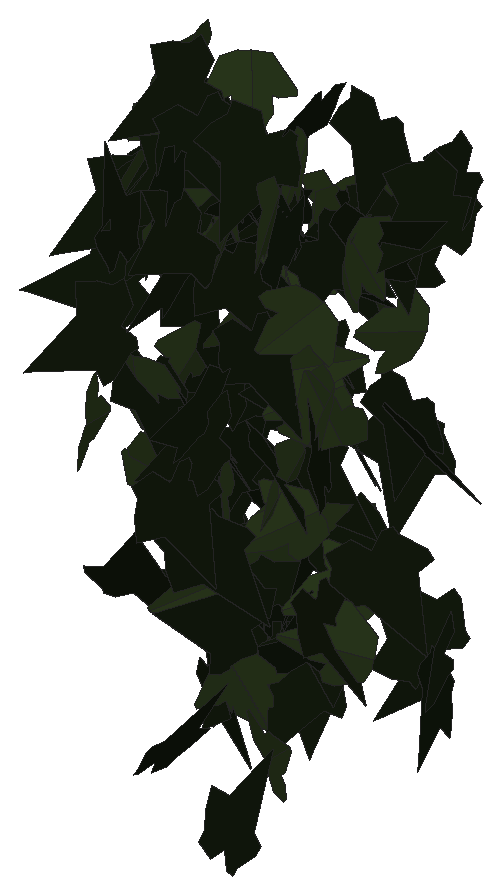
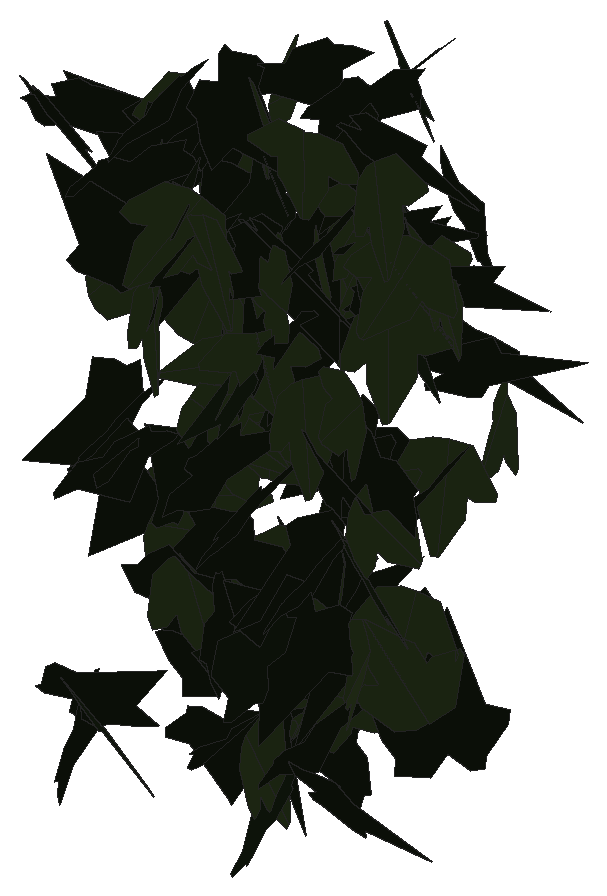
# SketchUp Ruby script. Lengths in inches.
U = 1.inch
M = Sketchup.active_model
def pt(a) = Geom::Point3d.new(a.map { |v| v * U })
def face(e, loops, mat)
  f = e.add_face(loops[0].map { |a| pt(a) })
  loops[1..].each { |l| e.add_face(l.map { |a| pt(a) }).erase! }
  f.material = f.back_material = mat if mat
  f
end
# faces: each face lists its corners as indices into pts; further lists are holes
def faces(e, pts, list, mat = nil) = list.each { |f| face(e, (f[0].is_a?(Array) ? f : [f]).map { |l| l.map { |i| pts[i] } }, mat) }
# xy, xz, yz: faces in a plane at the given z, y or x. An outline is a flat list of corners, or four numbers for a rectangle; further outlines are holes
def ring(l) = l.size == 4 ? [[l[0], l[1]], [l[2], l[1]], [l[2], l[3]], [l[0], l[3]]] : l.each_slice(2).to_a
def flat(e, list, mat, &to3) = list.each { |f| face(e, (f[0].is_a?(Array) ? f : [f]).map { |l| ring(l).map { |u, v| to3.(u, v) } }, mat) }
def xy(e, z, list, mat = nil) = flat(e, list, mat) { |x, y| [x, y, z] }
def xz(e, y, list, mat = nil) = flat(e, list, mat) { |x, z| [x, y, z] }
def yz(e, x, list, mat = nil) = flat(e, list, mat) { |y, z| [x, y, z] }
def lines(e, pts, list) = list.each { |a, b| e.add_line(pt(pts[a]), pt(pts[b])) }
# prism: a flat outline (further loops are holes) pulled along v
def prism(e, loops, v, mat = nil)
  f = face(e, loops, mat); d = Geom::Vector3d.new(v.map { |x| x * U })
  f.pushpull(f.normal.samedirection?(d) ? d.length : -d.length)
end
def box(e, o, s, mat = nil) = prism(e, [[o, [o[0] + s[0], o[1], o[2]], [o[0] + s[0], o[1] + s[1], o[2]], [o[0], o[1] + s[1], o[2]]]], [0, 0, s[2]], mat)
def at(x, y, z, deg = 0) = Geom::Transformation.translation(pt([x, y, z])) * Geom::Transformation.rotation(ORIGIN, Z_AXIS, deg.degrees)
def axes(o, x, y, z) = Geom::Transformation.new([*x, 0, *y, 0, *z, 0, *pt(o).to_a, 1])
def part(name) = M.definitions.add(name)
# library, detail: a bought-in or finely detailed component or shape, given as its bounding box
def library(name, o, s) = part(name).tap { |d| box(d.entities, o, s) }
def detail(e, o, s) = box(e.add_group.entities, o, s)
def put(e, d, t, mat = nil) = e.add_instance(d, t).tap { |i| i.material = mat if mat }
def group(e, t, mat = nil) = e.add_group.tap { |g| g.transformation = t; g.material = mat if mat }.entities
root = M.entities
M.materials.add("efeu1").color = [18, 25, 13]
M.materials.add("efeu2").color = [43, 57, 29]
c1 = part("ivyleaf_9")
p = [[1.54,2.16,1.25],[1.36,2.04,1.19],[-0.21,0.99,0.68],[-0.71,1.11,0.82],[-0.85,0.86,0.67],[-0.8,0.17,0.21],
  [-0.9,-0.01,0.1],[-0.67,-0.16,-0.02],[-0.08,-0.08,-0.05],[-0.03,-0.6,-0.4],[0.65,-0.88,-0.66],[0.83,-0.6,-0.49],
  [1.29,-0.42,-0.43],[1.8125,-0.07,-0.26],[1.21,0.44,0.15]]
faces(c1.entities,p,[[0,1,2,3,4,5,6,7,8,9,10,11,12,13,14]],"efeu1")
c2 = part("ivyleaf_10")
p = [[0,0.5,-0.03],[-0.0625,2.02,-0.43],[-0.19,2.01,-0.46],[-0.54,1.05,-0.29],[-0.52,0.625,-0.18],[-0.83,0.76,-0.28],
  [-1.16,0.64,-0.33],[-1.15,0.33,-0.24],[-0.77,-0.39,0.02],[-0.3,-0.51,0.16],[0.04,-0.48,0.23],[-0.02,2.01,-0.4375],
  [-0.06,2.01,-0.43],[0.04,-0.49,0.23],[0.67,-0.49,0.14],[1.38,0.36,-0.2],[1.375,0.51,-0.24],[0.81,0.65,-0.19],
  [0.62,0.59,-0.15],[0.6,1.09,-0.28],[0.5,1.23,-0.31]]
faces(c2.entities,p,[[0,1,2,3,4,5,6,7,8,9,10],[11,12,0,13,14,15,16,17,18,19,20]],"efeu2")
put(root,c1,axes([44.17,216.95,233.36],[-0.29201,0.31391,0.25727],[0.16965,-0.19353,0.42868],[0.36872,0.33765,0.00651]))
put(root,c1,axes([43.1875,217.07,238.26],[0.09081,-0.40776,-0.27475],[-0.05016,0.27025,-0.41767],[0.48912,0.10342,0.00818]))
put(root,c1,axes([43.4,217.47,239.27],[-0.33404,0.36237,0.08429],[-0.06458,0.05508,-0.49274],[-0.3664,-0.34008,0.01001]))
put(root,c1,axes([43.44,217.63,238.82],[-0.46053,0.16691,0.10026],[-0.09211,0.04007,-0.48981],[-0.17154,-0.46961,-0.00615]))
put(root,c1,axes([42.54,217.61,233.78],[0.12144,0.48134,0.0597],[-0.01468,-0.05787,0.49642],[0.48481,-0.12232,0.00007]))
put(root,c1,axes([42.3,218.62,241.02],[-0.23644,-0.26405,0.35267],[-0.0424,-0.38475,-0.3165],[0.43852,-0.17957,0.15955]))
put(root,c1,axes([42.65,218.31,236.78],[-0.0992,-0.12338,-0.47427],[0.29676,0.36996,-0.15831],[0.38999,-0.3129,-0.00017]))
put(root,c1,axes([41.8125,218.78,241.72],[-0.30616,0.00311,-0.3953],[0.38456,-0.11348,-0.29873],[-0.09157,-0.48694,0.06709]))
put(root,c2,axes([43.38,218.8,233.52],[-0.31281,0.08218,0.38131],[0.36576,-0.10801,0.32334],[0.13552,0.48123,0.00746]))
put(root,c2,axes([44.71,218.92,235.52],[0.06726,0.05582,0.4923],[-0.38955,-0.30103,0.08735],[0.30615,-0.3953,0.003]))
put(root,c2,axes([40.68,218.45,237.75],[0.03733,-0.19459,-0.45906],[-0.06731,0.45417,-0.19799],[0.49404,0.07658,0.00771]))
put(root,c1,axes([44.1875,218.84,236.09],[0.26012,-0.38428,-0.18619],[-0.10089,0.15654,-0.46402],[0.41492,0.27898,0.0039]))
put(root,c1,axes([40.67,219.06,238.86],[-0.47798,0.04874,0.13844],[-0.13878,0.00338,-0.48034],[-0.04776,-0.49761,0.01029]))
put(root,c1,axes([41.76,219.1,240.16],[-0.39385,0.2937,-0.09287],[0.07562,-0.05394,-0.4913],[-0.29861,-0.40104,-0.00193]))
put(root,c1,axes([42.52,219.4375,234.9],[-0.07693,-0.05425,0.49106],[-0.3839,-0.30625,-0.09398],[0.31097,-0.39149,0.00547]))
put(root,c1,axes([40.82,218.93,240.1875],[0.08447,0.03015,0.49189],[-0.20318,0.4568,0.00689],[-0.44898,-0.20105,0.08942]))
put(root,c2,axes([42.86,219.51,241.18],[0.05398,-0.15015,0.47386],[0.30302,-0.3679,-0.15109],[0.39404,0.30349,0.05128]))
put(root,c2,axes([43.4375,219.42,236.86],[-0.18949,-0.12269,0.44614],[-0.2797,-0.35368,-0.21605],[0.3686,-0.33145,0.0654]))
put(root,c1,axes([42.73,219.3,239.34],[-0.17253,-0.1136,-0.45533],[0.37118,0.26382,-0.20646],[0.28716,-0.40926,-0.0067]))
put(root,c2,axes([43.58,219.37,239.95],[0.36612,0.07803,-0.33146],[-0.33824,0.02713,-0.36723],[-0.03933,0.49313,0.07266]))
put(root,c2,axes([43.04,219.73,237.35],[0.08516,-0.18325,0.45735],[0.2054,-0.40867,-0.202],[0.44784,0.22228,0.00567]))
put(root,c2,axes([42.52,219.28,234.26],[-0.32308,-0.33079,-0.19025],[0.1444,0.12477,-0.46215],[0.35323,-0.35356,0.01491]))
put(root,c1,axes([43.84,219.36,237.59],[0.09451,-0.36638,0.32686],[0.04105,0.33759,0.36653],[-0.48927,-0.04245,0.0939]))
put(root,c1,axes([42.8,219.68,237.4],[0.15539,-0.3737,0.2936],[0.1732,-0.24313,-0.40111],[0.44256,0.22636,0.05389]))
put(root,c2,axes([43.88,219.54,238.23],[-0.43634,-0.16803,-0.17712],[-0.16603,-0.06174,0.46757],[-0.17901,0.46685,-0.00191]))
put(root,c2,axes([43.81,219.42,238.79],[0.32451,-0.34146,-0.16763],[-0.11759,0.1195,-0.47105],[0.36175,0.34515,-0.00275]))
put(root,c1,axes([41.76,219.63,233.9],[-0.0089,0.01269,-0.49976],[0.499,0.03056,-0.00811],[0.03033,-0.4989,-0.0132]))
put(root,c1,axes([42.46,219.86,241.93],[-0.27279,-0.41886,0.01203],[-0.00827,-0.00898,-0.49985],[0.41895,-0.27291,-0.00203]))
put(root,c1,axes([40.26,219.91,239.02],[-0.33135,-0.04916,0.3712],[-0.33074,-0.19397,-0.32092],[0.17556,-0.45821,0.09602]))
put(root,c2,axes([43.96,219.93,235.82],[-0.18203,0.01179,0.46554],[-0.23954,-0.43102,-0.08274],[0.39936,-0.25315,0.16256]))
put(root,c1,axes([41.49,219.73,241.91],[0.0202,-0.39898,-0.30068],[0.0152,0.30128,-0.39875],[0.49936,0.00697,0.0243]))
put(root,c1,axes([40.3,219.89,234.48],[0.47165,0.05631,0.15613],[-0.15478,-0.02058,0.475],[0.05992,-0.49639,-0.00198]))
put(root,c1,axes([43.16,219.89,234.47],[0.38109,0.21726,0.23993],[-0.2205,-0.09709,0.43813],[0.23696,-0.43974,0.02181]))
put(root,c1,axes([41.52,219.65,237.61],[0.45763,-0.04302,-0.19678],[-0.19307,0.04556,-0.45896],[0.05742,0.49606,0.02509]))
put(root,c1,axes([42.125,220.24,233.93],[-0.17309,-0.36371,0.29623],[-0.08076,-0.28793,-0.40071],[0.46208,-0.18657,0.04093]))
put(root,c2,axes([40.41,219.82,237.83],[-0.49301,-0.07431,0.03763],[-0.03669,-0.00909,-0.49857],[0.07479,-0.49436,0.00351]))
put(root,c1,axes([43.02,219.55,240.46],[-0.01399,0.16256,0.47263],[-0.16266,0.4456,-0.15807],[-0.4726,-0.15818,0.04041]))
put(root,c1,axes([40.29,220.17,240.17],[-0.40828,-0.20075,0.20738],[-0.15858,-0.14415,-0.45174],[0.24117,-0.43465,0.05404]))
put(root,c2,axes([41.58,220.13,236.375],[-0.17197,0.17532,-0.43554],[0.20308,-0.39042,-0.23734],[-0.4233,-0.25852,0.06307]))
put(root,c1,axes([40.4,220.09,237.64],[0.11712,-0.48603,-0.00796],[-0.00042,0.00808,-0.49993],[0.48609,0.11711,0.00148]))
put(root,c2,axes([44.125,219.74,240.92],[-0.0946,0.42249,0.2501],[-0.09576,0.23393,-0.4314],[-0.48154,-0.12952,0.03665]))
put(root,c1,axes([44.17,219.99,236.31],[-0.08439,-0.30346,-0.38832],[0.2181,0.33029,-0.30552],[0.44194,-0.22095,0.07662]))
put(root,c1,axes([40.95,220.37,240.6],[-0.34879,-0.23503,0.27038],[-0.16878,-0.22506,-0.41336],[0.31601,-0.37962,0.07766]))
put(root,c2,axes([40.98,219.81,240.24],[-0.15524,-0.31879,-0.35252],[0.23607,0.27015,-0.34826],[0.41252,-0.27457,0.06664]))
put(root,c2,axes([44.05,219.6875,240.66],[-0.06117,0.21059,0.44935],[-0.27302,0.36379,-0.20765],[-0.41439,-0.27076,0.07049]))
put(root,c2,axes([41.49,220.25,234.875],[0.14082,0.14904,-0.45602],[-0.39655,-0.23134,-0.19807],[-0.27003,0.41745,0.05305]))
put(root,c1,axes([41.32,219.95,241.375],[0.47809,-0.07001,-0.12857],[-0.12677,0.02164,-0.48318],[0.07322,0.4946,0.00294]))
put(root,c2,axes([41.59,220.26,240.29],[0.14256,-0.4602,0.13378],[0.0301,-0.1307,-0.48168],[0.4783,0.14539,-0.00956]))
put(root,c1,axes([43.43,219.85,240.74],[0.1524,-0.17094,-0.44447],[-0.14093,0.42958,-0.21354],[0.45488,0.19036,0.08276]))
put(root,c1,axes([42.76,220.47,233.98],[-0.2178,-0.43133,0.12852],[-0.00011,-0.14273,-0.4792],[0.45007,-0.20876,0.06207]))
put(root,c2,axes([40.45,220.23,240.69],[0.40656,-0.28415,0.06299],[0.05167,-0.03603,-0.49602],[0.28643,0.40983,0.00007]))
put(root,c2,axes([42.7,220.36,239.27],[0.10063,-0.45376,0.18433],[0.02622,-0.18291,-0.4646],[0.48907,0.10317,-0.01302]))
put(root,c2,axes([42.76,220.18,241.68],[0.36785,-0.32655,-0.0897],[-0.05342,0.07483,-0.49147],[0.33441,0.37117,0.02017]))
put(root,c2,axes([42.33,219.97,236.07],[-0.23647,-0.24217,-0.36802],[0.24327,0.27645,-0.33822],[0.36729,-0.33901,-0.01292]))
put(root,c1,axes([40.49,220.55,240.29],[-0.31565,-0.38671,0.02865],[-0.0178,-0.02246,-0.49918],[0.38736,-0.31615,0.00042]))
put(root,c2,axes([40,220.42,240.53],[0.15917,-0.47138,0.04967],[0.01528,-0.04726,-0.49753],[0.47374,0.1599,-0.00065]))
put(root,c1,axes([40.9,220.48,241.92],[-0.49003,-0.00936,0.09889],[-0.0986,-0.01438,-0.48997],[0.01202,-0.49971,0.01225]))
put(root,c1,axes([43.73,220.29,240.49],[0.01571,-0.09515,0.49061],[0.48872,-0.09964,-0.03497],[0.10443,0.48064,0.08987]))
put(root,c1,axes([42.05,220.65,235.26],[-0.43503,-0.24229,0.04517],[-0.04097,-0.01927,-0.49795],[0.24304,-0.43695,-0.00309]))
put(root,c1,axes([42.67,220.3125,240.1],[0.4275,-0.05709,0.25295],[0.249,-0.04579,-0.43116],[0.07239,0.49462,-0.01072]))
put(root,c1,axes([42.13,220.4,240.72],[0.44565,-0.22128,0.04925],[0.04367,-0.02279,-0.49757],[0.22245,0.44779,-0.00099]))
put(root,c1,axes([42.74,220.56,234.21],[-0.29414,-0.32896,-0.23509],[0.14938,0.18174,-0.4412],[0.37572,-0.32979,-0.00864]))
put(root,c1,axes([40.85,220.37,240.16],[-0.32289,0.38042,-0.03191],[0.02019,-0.02473,-0.49898],[-0.38122,-0.32352,0.00061]))
put(root,c2,axes([41.11,220.45,240.78],[-0.4075,0.21224,-0.19723],[0.1653,-0.10922,-0.45907],[-0.23795,-0.43935,0.01884]))
put(root,c2,axes([42.71,220.15,238.43],[0.00134,-0.03376,0.49886],[0.1628,0.4717,0.03149],[-0.47275,0.16235,0.01225]))
put(root,c2,axes([40.375,220.47,236.31],[-0.49363,-0.06856,-0.04031],[0.04018,0.00373,-0.49837],[0.06863,-0.49526,0.00183]))
put(root,c2,axes([44.05,220.87,239.19],[-0.01322,0.19339,0.4609],[0.05102,-0.45813,0.19369],[0.49721,0.05215,-0.00762]))
put(root,c2,axes([40.7,220.43,240.07],[-0.34681,0.08061,0.35104],[-0.347,0.05582,-0.35563],[-0.09652,-0.49029,0.01722]))
put(root,c1,axes([41.11,220.44,235.73],[0.15677,-0.32778,-0.34349],[-0.15226,0.30792,-0.36332],[0.44971,0.21851,-0.00327]))
put(root,c2,axes([42.85,220.73,237.95],[-0.24859,0.00617,0.43378],[-0.37312,-0.25809,-0.21016],[0.22132,-0.42819,0.13292]))
put(root,c1,axes([41.49,220.25,236.69],[0.07045,0.01906,-0.49464],[-0.13744,0.48074,-0.00105],[0.47555,0.13611,0.07298]))
put(root,c2,axes([42.23,220.97,238.59],[0.05508,0.16523,-0.46868],[-0.13327,-0.44937,-0.17409],[-0.47875,0.1441,-0.00546]))
put(root,c1,axes([41.4,220.59,239.47],[0.01739,-0.36795,-0.33809],[-0.02266,0.33737,-0.36833],[0.49918,0.02814,-0.00495]))
put(root,c1,axes([42.59,220.82,242.04],[-0.22735,0.2606,-0.36111],[0.18797,-0.31141,-0.34306],[-0.40371,-0.29175,0.04363]))
put(root,c1,axes([42.53,220.97,235.78],[-0.1274,0.03761,-0.48203],[0.37614,-0.3055,-0.12325],[-0.30379,-0.39402,0.04955]))
put(root,c1,axes([41.82,220.66,240.45],[0.064,0.38027,-0.31827],[-0.10249,-0.30384,-0.38364],[-0.48518,0.11434,0.03906]))
put(root,c2,axes([40.46,220.97,237.71],[-0.01193,-0.38616,0.31739],[0.02091,-0.31759,-0.38562],[0.49942,0.00408,0.02373]))
put(root,c1,axes([42.1,220.99,238.74],[-0.01282,-0.07901,0.49355],[0.12935,-0.47742,-0.07307],[0.48281,0.12581,0.03268]))
put(root,c1,axes([41.53,220.57,237.69],[-0.33788,0.0425,-0.36611],[-0.368,-0.01142,0.3383],[0.0204,0.49806,0.039]))
put(root,c1,axes([43.34,220.8,235.5625],[-0.14754,0.05781,0.47423],[-0.46365,0.10232,-0.15672],[-0.11516,-0.48599,0.02342]))
put(root,c1,axes([42.08,220.59,234.63],[0.06388,-0.00337,-0.49589],[-0.49571,0.0136,-0.06395],[0.01392,0.4998,-0.0016]))
put(root,c1,axes([42.92,221.02,237.24],[0.16407,-0.2583,0.39543],[0.19077,-0.3467,-0.30563],[0.43207,0.25116,-0.01521]))
put(root,c2,axes([40.31,220.45,240.09],[0.14963,0.23983,0.41242],[0.11632,0.40085,-0.2753],[-0.46269,0.17833,0.06417]))
put(root,c1,axes([44.57,221.03,241.29],[-0.44056,-0.22312,0.07825],[-0.06274,-0.04924,-0.4936],[0.22797,-0.44474,0.01539]))
put(root,c2,axes([41.49,220.78,238.58],[-0.1072,-0.4865,-0.0427],[0.00966,0.0416,-0.49817],[0.48828,-0.10764,0.00048]))
put(root,c1,axes([40.59,220.66,240.72],[-0.33262,0.29628,0.22711],[-0.16168,0.15984,-0.44532],[-0.33648,-0.36969,-0.01053]))
put(root,c2,axes([42.96,220.9,236.05],[-0.22557,-0.43236,0.11037],[-0.05582,-0.09535,-0.48764],[0.44272,-0.23232,-0.00525]))
put(root,c2,axes([40,220.79,235.54],[-0.34839,-0.24197,0.26472],[0.21349,0.15663,0.42413],[-0.28818,0.40856,-0.00582]))
put(root,c1,axes([42.26,220.76,236.65],[0.04459,-0.17189,-0.4674],[0.32554,0.36519,-0.10325],[0.37688,-0.29511,0.14449]))
put(root,c1,axes([43.04,221.2,240.22],[0.06911,-0.30735,0.38828],[0.0937,-0.37684,-0.31498],[0.48625,0.1163,0.00551]))
put(root,c1,axes([41.88,220.99,240.55],[-0.49324,0.08193,-0.00144],[0.00158,0.00071,-0.5],[-0.08192,-0.49324,-0.00096]))
put(root,c1,axes([43.6,221.08,240.86],[-0.07832,-0.45421,-0.19381],[0.04936,0.18805,-0.46065],[0.49135,-0.09129,0.01538]))
put(root,c1,axes([42.77,220.93,240.12],[0.16787,-0.37741,-0.28175],[-0.10507,0.26157,-0.41297],[0.45911,0.19786,0.00851]))
put(root,c1,axes([43.8125,220.97,237.69],[0.44602,-0.18357,0.1318],[0.12153,-0.05103,-0.48231],[0.19053,0.46227,-0.00091]))
put(root,c1,axes([44.18,221.3,233.95],[0.04336,-0.01409,-0.49792],[0.40918,-0.28402,0.04367],[-0.28407,-0.41126,-0.01311]))
put(root,c1,axes([43.17,221.35,241.73],[-0.01011,-0.46904,0.17291],[-0.00918,-0.17274,-0.46912],[0.49981,-0.01266,-0.00512]))
put(root,c1,axes([40.25,221.11,238.5],[-0.2052,-0.08752,-0.44748],[0.42129,0.15128,-0.22277],[0.17438,-0.46846,0.01166]))
put(root,c2,axes([40.18,221.03,240.0625],[-0.25402,-0.42964,-0.02975],[0.01184,0.02755,-0.4991],[0.4305,-0.25427,-0.00382]))
put(root,c1,axes([43.67,221.37,237.76],[-0.00725,-0.46673,0.1792],[0.0092,-0.17931,-0.46665],[0.49986,-0.00347,0.01119]))
put(root,c2,axes([41.83,221.11,239.3],[0.39544,0.29731,-0.07233],[-0.05025,-0.05348,-0.49459],[-0.30183,0.39843,-0.01242]))
put(root,c1,axes([43.74,221.34,237.39],[-0.13185,-0.48228,0.00417],[0.00225,-0.00494,-0.49997],[0.4823,-0.13182,0.00347]))
put(root,c1,axes([40.74,221.33,241.15],[0.0758,-0.48725,0.08273],[0.02565,-0.0797,-0.49294],[0.49356,0.07897,0.01291]))
put(root,c2,axes([41.49,221.22,240],[-0.00844,-0.04616,0.49779],[0.48986,-0.10016,-0.00098],[0.09981,0.48769,0.04691]))
put(root,c1,axes([41.03,221.36,234.94],[-0.02649,-0.49503,0.06514],[-0.00655,-0.06488,-0.49573],[0.49925,-0.02712,-0.00305]))
put(root,c2,axes([39.91,221.02,240.94],[-0.39797,-0.20296,-0.22456],[0.22475,0.05033,-0.4438],[0.20275,-0.45418,0.05117]))
put(root,c2,axes([41.21,221.12,241.9375],[0.4764,0.12906,0.07989],[0.07452,0.03039,-0.49348],[-0.13223,0.4821,0.00972]))
put(root,c1,axes([41.96,221.12,238.93],[0.37682,-0.32497,-0.04896],[-0.02973,0.04046,-0.49747],[0.32729,0.37783,0.01117]))
put(root,c1,axes([44.33,221.17,234.36],[-0.45291,0.20802,-0.03999],[0.03593,-0.01759,-0.4984],[-0.20876,-0.45433,0.00098]))
put(root,c2,axes([41.7,221.32,234.53],[0.11056,-0.454,0.17794],[0.05102,-0.17068,-0.46719],[0.48495,0.12146,0.00859]))
put(root,c1,axes([41.98,221.53,237.2],[0.15044,-0.4121,-0.23989],[0.07661,-0.22739,0.43866],[-0.47064,-0.16874,-0.00527]))
put(root,c1,axes([41.27,220.96,236.18],[0.41688,0.24354,-0.13],[-0.11433,-0.06201,-0.48279],[-0.25128,0.43225,0.00399]))
put(root,c1,axes([40.97,221.16,234.23],[-0.34799,0.20207,0.29677],[-0.29033,0.08475,-0.39815],[-0.21121,-0.44943,0.05835]))
put(root,c2,axes([40.14,221.23,241.88],[0.00427,-0.498,-0.04446],[0.00598,0.04451,-0.49798],[0.49995,0.00372,0.00633]))
put(root,c2,axes([40.34,221.3125,236.14],[-0.24569,0.34388,-0.26718],[0.14503,-0.22464,-0.4225],[-0.41061,-0.2851,0.01064]))
put(root,c2,axes([42.49,221.24,240.41],[-0.45052,0.13496,0.16975],[-0.20039,-0.10946,-0.44482],[-0.0829,-0.46883,0.15272]))
put(root,c1,axes([41.44,221.54,233.83],[0.11355,-0.3829,0.30082],[0.07971,-0.29011,-0.39935],[0.48037,0.13865,-0.00485]))
put(root,c1,axes([40.4,221.38,237.41],[-0.41901,0.09193,-0.25687],[0.24623,-0.0753,-0.4286],[-0.11749,-0.48567,0.01783]))
put(root,c1,axes([40.9,221.52,236.98],[0.05719,-0.48074,0.12499],[-0.0025,-0.12609,-0.48383],[0.49671,0.05472,-0.01683]))
put(root,c1,axes([42.24,221.67,237.87],[0.06687,-0.3124,-0.38463],[0.07852,-0.37653,0.31947],[-0.48925,-0.10313,-0.0013]))
put(root,c1,axes([44.51,221.4,241.4375],[-0.47985,0.08031,-0.11529],[0.11309,-0.02268,-0.48651],[-0.08338,-0.49299,0.0036]))
put(root,c1,axes([43.42,221.25,239.85],[-0.14665,0.00501,0.47798],[0.4581,-0.14133,0.14203],[0.13653,0.47958,0.03686]))
put(root,c1,axes([44.13,221.33,234.36],[-0.41522,-0.23004,-0.15708],[-0.13757,-0.07582,0.47469],[-0.24221,0.43742,-0.00033]))
put(root,c1,axes([41.5,221.47,235.74],[0.29115,-0.30754,0.26581],[0.19272,-0.18344,-0.42333],[0.3579,0.34896,0.01172]))
put(root,c2,axes([42.76,221.22,240.6],[-0.39001,-0.16107,-0.26823],[0.24804,0.1021,-0.42196],[0.19071,-0.4622,0.00026]))
put(root,c2,axes([40.37,221.45,239.2],[-0.31403,0.20045,-0.33348],[0.24028,-0.23715,-0.36882],[-0.30602,-0.39189,0.05262]))
put(root,c2,axes([43.31,221.16,239.37],[-0.30857,0.17635,0.35169],[-0.31797,0.15142,-0.35492],[-0.23169,-0.44269,0.0187]))
